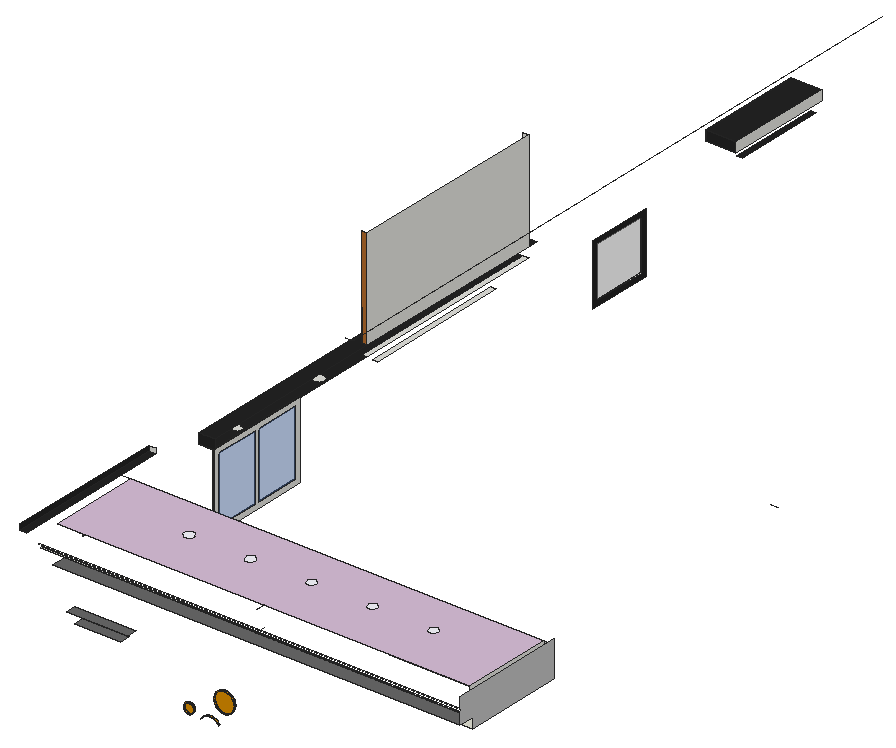
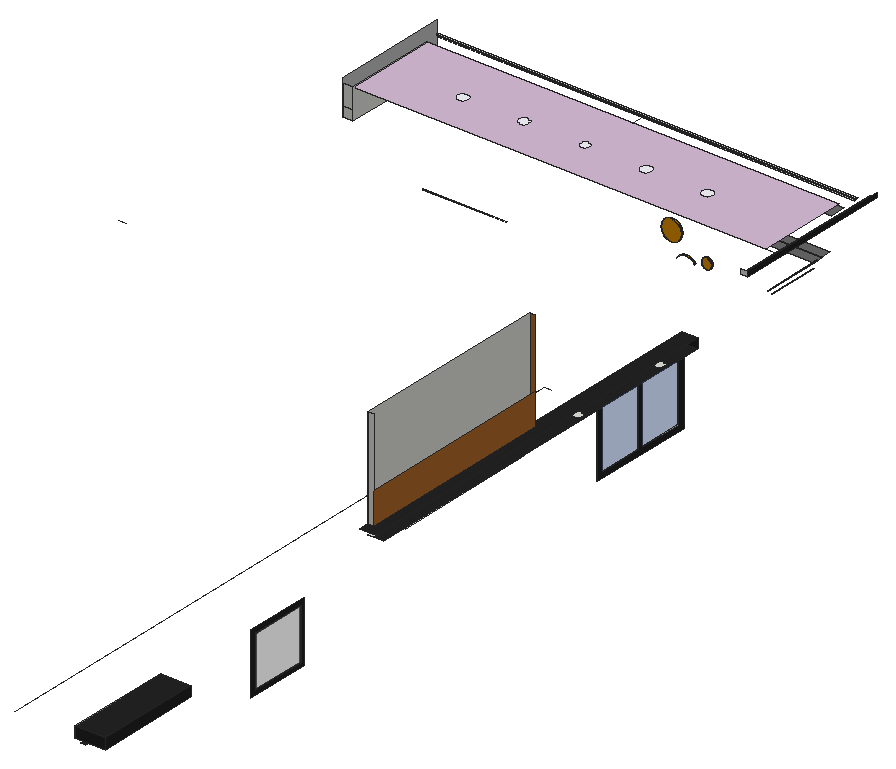
# SketchUp Ruby script. Lengths in inches.
U = 1.inch
M = Sketchup.active_model
def pt(a) = Geom::Point3d.new(a.map { |v| v * U })
def face(e, loops, mat)
  f = e.add_face(loops[0].map { |a| pt(a) })
  loops[1..].each { |l| e.add_face(l.map { |a| pt(a) }).erase! }
  f.material = f.back_material = mat if mat
  f
end
# faces: each face lists its corners as indices into pts; further lists are holes
def faces(e, pts, list, mat = nil) = list.each { |f| face(e, (f[0].is_a?(Array) ? f : [f]).map { |l| l.map { |i| pts[i] } }, mat) }
# xy, xz, yz: faces in a plane at the given z, y or x. An outline is a flat list of corners, or four numbers for a rectangle; further outlines are holes
def ring(l) = l.size == 4 ? [[l[0], l[1]], [l[2], l[1]], [l[2], l[3]], [l[0], l[3]]] : l.each_slice(2).to_a
def flat(e, list, mat, &to3) = list.each { |f| face(e, (f[0].is_a?(Array) ? f : [f]).map { |l| ring(l).map { |u, v| to3.(u, v) } }, mat) }
def xy(e, z, list, mat = nil) = flat(e, list, mat) { |x, y| [x, y, z] }
def xz(e, y, list, mat = nil) = flat(e, list, mat) { |x, z| [x, y, z] }
def yz(e, x, list, mat = nil) = flat(e, list, mat) { |y, z| [x, y, z] }
def lines(e, pts, list) = list.each { |a, b| e.add_line(pt(pts[a]), pt(pts[b])) }
# prism: a flat outline (further loops are holes) pulled along v
def prism(e, loops, v, mat = nil)
  f = face(e, loops, mat); d = Geom::Vector3d.new(v.map { |x| x * U })
  f.pushpull(f.normal.samedirection?(d) ? d.length : -d.length)
end
def box(e, o, s, mat = nil) = prism(e, [[o, [o[0] + s[0], o[1], o[2]], [o[0] + s[0], o[1] + s[1], o[2]], [o[0], o[1] + s[1], o[2]]]], [0, 0, s[2]], mat)
def at(x, y, z, deg = 0) = Geom::Transformation.translation(pt([x, y, z])) * Geom::Transformation.rotation(ORIGIN, Z_AXIS, deg.degrees)
def axes(o, x, y, z) = Geom::Transformation.new([*x, 0, *y, 0, *z, 0, *pt(o).to_a, 1])
def part(name) = M.definitions.add(name)
# library, detail: a bought-in or finely detailed component or shape, given as its bounding box
def library(name, o, s) = part(name).tap { |d| box(d.entities, o, s) }
def detail(e, o, s) = box(e.add_group.entities, o, s)
def put(e, d, t, mat = nil) = e.add_instance(d, t).tap { |i| i.material = mat if mat }
def group(e, t, mat = nil) = e.add_group.tap { |g| g.transformation = t; g.material = mat if mat }.entities
root = M.entities
M.materials.add("[0038_Orange]").color = [221, 143, 0]
M.materials.add("[0053_Ivory]").color = [255, 255, 240]
M.materials.add("[0117_GhostWhite]").color = [248, 248, 255]
M.materials.add("[0118_Thistle]").color = [216, 191, 216]
M.materials.add("[0131_Silver]").color = [192, 192, 192]
M.materials.add("[0134_DimGray]").color = [105, 105, 105]
M.materials.add("[0135_DarkGray]").color = [35, 35, 35]
M.materials.add("[Translucent Glass Blue]").color = [73, 109, 173]
M.materials["[Translucent Glass Blue]"].alpha = 0.5
M.materials.add("[Translucent Glass Gray]").color = [163, 163, 163]
M.materials["[Translucent Glass Gray]"].alpha = 0.5
M.materials.add("[Wood Bamboo]").color = [177, 105, 43]
xy(root,735.4,[[70,1678.125,72,1810.125]])
xy(root,735.4,[[69,552,72,804]],"[0135_DarkGray]")
xy(root,744.7,[[513.45,27,515.96,30]],"[0038_Orange]")
xy(root,747.4,[[69,564,72,673],[69,683,72,792]],"[0135_DarkGray]")
xy(root,822,[[174,12,282,36]],"[0134_DimGray]")
xy(root,827.4375,[[705.53,276,902.41,278]])
xy(root,840,[[156,12,300,36]],"[0134_DimGray]")
xy(root,849.4,[[60,2106,72,2322]],"[0135_DarkGray]")
xy(root,855.4,[[70,1678.125,72,1810.125]])
xy(root,867.4,[[60,2088,72,2340],[30,2202,28.75,2202.07,27.51,2202.26,26.29,2202.59,25.12,2203.04,24,2203.61,22.95,2204.29,21.97,2205.08,21.08,2205.97,20.29,2206.95,19.61,2208,19.04,2209.12,18.59,2210.29,18.26,2211.51,18.07,2212.75,18,2214,18.07,2215.25,18.26,2216.49,18.59,2217.71,19.04,2218.88,19.61,2220,20.29,2221.05,21.08,2222.03,21.97,2222.92,22.95,2223.71,24,2224.39,25.12,2224.96,26.29,2225.41,27.51,2225.74,28.75,2225.93,30,2226,31.25,2225.93,32.49,2225.74,33.71,2225.41,34.88,2224.96,36,2224.39,37.05,2223.71,38.03,2222.92,38.92,2222.03,39.71,2221.05,40.39,2220,40.96,2218.88,41.41,2217.71,41.74,2216.49,41.93,2215.25,42,2214,41.93,2212.75,41.74,2211.51,41.41,2210.29,40.96,2209.12,40.39,2208,39.71,2206.95,38.92,2205.97,38.03,2205.08,37.05,2204.29,36,2203.61,34.88,2203.04,33.71,2202.59,32.49,2202.26,31.25,2202.07]])
xy(root,867.4,[[[0,2088,60,2340],[30,2202,31.25,2202.07,32.49,2202.26,33.71,2202.59,34.88,2203.04,36,2203.61,37.05,2204.29,38.03,2205.08,38.92,2205.97,39.71,2206.95,40.39,2208,40.96,2209.12,41.41,2210.29,41.74,2211.51,41.93,2212.75,42,2214,41.93,2215.25,41.74,2216.49,41.41,2217.71,40.96,2218.88,40.39,2220,39.71,2221.05,38.92,2222.03,38.03,2222.92,37.05,2223.71,36,2224.39,34.88,2224.96,33.71,2225.41,32.49,2225.74,31.25,2225.93,30,2226,28.75,2225.93,27.51,2225.74,26.29,2225.41,25.12,2224.96,24,2224.39,22.95,2223.71,21.97,2222.92,21.08,2222.03,20.29,2221.05,19.61,2220,19.04,2218.88,18.59,2217.71,18.26,2216.49,18.07,2215.25,18,2214,18.07,2212.75,18.26,2211.51,18.59,2210.29,19.04,2209.12,19.61,2208,20.29,2206.95,21.08,2205.97,21.97,2205.08,22.95,2204.29,24,2203.61,25.12,2203.04,26.29,2202.59,27.51,2202.26,28.75,2202.07]]],"[0135_DarkGray]")
xy(root,891.4,[[60,1032,72,1380]])
xy(root,891.4,[[0,2088,72,2340]],"[0135_DarkGray]")
xy(root,903.4,[[69,167.11,72,287.92],[69,564,72,673],[69,683,72,792]],"[0135_DarkGray]")
xy(root,912,[[582,36,582,60,1068,60,1068,276,1092,276,1092,36]])
xy(root,915.4,[[69,552,72,804],[52.84,630.27,51.59,630.38,50.36,630.62,49.16,630.99,48,631.48,46.9,632.09,45.875,632.81,44.93,633.64,44.07,634.56,43.32,635.56,42.67,636.64,42.14,637.78,41.74,638.97,41.46,640.19,41.31,641.44,41.29,642.7,41.4,643.95,41.64,645.18,42.01,646.38,42.5,647.54,43.11,648.63,43.83,649.66,44.66,650.61,45.58,651.46,46.58,652.22,47.66,652.86,48.8,653.39,49.99,653.8,51.21,654.08,52.46,654.23,53.72,654.25,54.97,654.14,56.2,653.9,57.4,653.53,58.55,653.04,59.65,652.43,60.68,651.7,61.625,650.88,62.48,649.96,63.24,648.95,63.88,647.875,64.41,646.74,64.82,645.55,65.1,644.32,65.25,643.08,65.27,641.82,65.16,640.57,64.92,639.34,64.55,638.14,64.05,636.98,63.44,635.88,62.72,634.86,61.9,633.91,60.98,633.05,59.97,632.3,58.89,631.66,57.76,631.125,56.57,630.72,55.34,630.4375,54.1,630.29],[52.84,870.64,51.59,870.75,50.36,871,49.16,871.36,48,871.86,46.9,872.47,45.875,873.19,44.93,874.02,44.07,874.94,43.32,875.94,42.67,877.02,42.14,878.16,41.74,879.34,41.46,880.57,41.31,881.82,41.29,883.07,41.4,884.32,41.64,885.56,42.01,886.76,42.5,887.91,43.11,889.01,43.83,890.04,44.66,890.98,45.58,891.84,46.58,892.59,47.66,893.24,48.8,893.77,49.99,894.17,51.21,894.46,52.46,894.61,53.72,894.625,54.97,894.51,56.2,894.27,57.4,893.9,58.55,893.41,59.65,892.8,60.68,892.08,61.625,891.25,62.48,890.33,63.24,889.33,63.88,888.25,64.41,887.11,64.82,885.92,65.1,884.7,65.25,883.45,65.27,882.2,65.16,880.95,64.92,879.71,64.55,878.51,64.05,877.36,63.44,876.26,62.72,875.23,61.9,874.28,60.98,873.43,59.97,872.68,58.89,872.03,57.76,871.5,56.57,871.09,55.34,870.8125,54.1,870.66],[60,1000.8,72,1476]])
xy(root,915.4,[[69,155.11,72,299.92],[[36,552,36,1476,60,1476,60,1000.8,72,1000.8,72,804,69,804,69,552],[52.84,870.64,54.1,870.66,55.34,870.8125,56.57,871.09,57.76,871.5,58.89,872.03,59.97,872.68,60.98,873.43,61.9,874.28,62.72,875.23,63.44,876.26,64.05,877.36,64.55,878.51,64.92,879.71,65.16,880.95,65.27,882.2,65.25,883.45,65.1,884.7,64.82,885.92,64.41,887.11,63.88,888.25,63.24,889.33,62.48,890.33,61.625,891.25,60.68,892.08,59.65,892.8,58.55,893.41,57.4,893.9,56.2,894.27,54.97,894.51,53.72,894.625,52.46,894.61,51.21,894.46,49.99,894.17,48.8,893.77,47.66,893.24,46.58,892.59,45.58,891.84,44.66,890.98,43.83,890.04,43.11,889.01,42.5,887.91,42.01,886.76,41.64,885.56,41.4,884.32,41.29,883.07,41.31,881.82,41.46,880.57,41.74,879.34,42.14,878.16,42.67,877.02,43.32,875.94,44.07,874.94,44.93,874.02,45.875,873.19,46.9,872.47,48,871.86,49.16,871.36,50.36,871,51.59,870.75],[52.84,630.27,54.1,630.29,55.34,630.4375,56.57,630.72,57.76,631.125,58.89,631.66,59.97,632.3,60.98,633.05,61.9,633.91,62.72,634.86,63.44,635.88,64.05,636.98,64.55,638.14,64.92,639.34,65.16,640.57,65.27,641.82,65.25,643.08,65.1,644.32,64.82,645.55,64.41,646.74,63.88,647.875,63.24,648.95,62.48,649.96,61.625,650.88,60.68,651.7,59.65,652.43,58.55,653.04,57.4,653.53,56.2,653.9,54.97,654.14,53.72,654.25,52.46,654.23,51.21,654.08,49.99,653.8,48.8,653.39,47.66,652.86,46.58,652.22,45.58,651.46,44.66,650.61,43.83,649.66,43.11,648.63,42.5,647.54,42.01,646.38,41.64,645.18,41.4,643.95,41.29,642.7,41.31,641.44,41.46,640.19,41.74,638.97,42.14,637.78,42.67,636.64,43.32,635.56,44.07,634.56,44.93,633.64,45.875,632.81,46.9,632.09,48,631.48,49.16,630.99,50.36,630.62,51.59,630.38]]],"[0135_DarkGray]")
xy(root,936,[[132,0,1092,36]],"[0134_DimGray]")
xy(root,939.4,[[60,1000.8,72,1476]])
xy(root,939.4,[[36,552,72,552,72,1000.8,60,1000.8,60,1476,72,1476,72,1500,36,1500]],"[0135_DarkGray]")
xy(root,963,[[105,0,1092,3]])
xy(root,969,[[99,0,1092,3]])
xy(root,984,[[310.43,167.36,307.32,167.77,304.43,168.97,301.94,170.88,300.04,173.36,298.84,176.26,298.43,179.36,298.84,182.47,300.04,185.36,301.94,187.85,304.43,189.75,307.32,190.95,310.43,191.36,313.53,190.95,316.43,189.75,318.91,187.85,320.82,185.36,322.02,182.47,322.43,179.36,322.02,176.26,320.82,173.36,318.91,170.88,316.43,168.97,313.53,167.77],[454.43,167.36,451.32,167.77,448.43,168.97,445.94,170.88,444.04,173.36,442.84,176.26,442.43,179.36,442.84,182.47,444.04,185.36,445.94,187.85,448.43,189.75,451.32,190.95,454.43,191.36,457.53,190.95,460.43,189.75,462.91,187.85,464.82,185.36,466.02,182.47,466.43,179.36,466.02,176.26,464.82,173.36,462.91,170.88,460.43,168.97,457.53,167.77],[598.43,167.36,595.32,167.77,592.43,168.97,589.94,170.88,588.04,173.36,586.84,176.26,586.43,179.36,586.84,182.47,588.04,185.36,589.94,187.85,592.43,189.75,595.32,190.95,598.43,191.36,601.53,190.95,604.43,189.75,606.91,187.85,608.82,185.36,610.02,182.47,610.43,179.36,610.02,176.26,608.82,173.36,606.91,170.88,604.43,168.97,601.53,167.77],[742.43,167.36,739.32,167.77,736.43,168.97,733.94,170.88,732.04,173.36,730.84,176.26,730.43,179.36,730.84,182.47,732.04,185.36,733.94,187.85,736.43,189.75,739.32,190.95,742.43,191.36,745.53,190.95,748.43,189.75,750.91,187.85,752.82,185.36,754.02,182.47,754.43,179.36,754.02,176.26,752.82,173.36,750.91,170.88,748.43,168.97,745.53,167.77],[886.43,167.36,883.32,167.77,880.43,168.97,877.94,170.88,876.04,173.36,874.84,176.26,874.43,179.36,874.84,182.47,876.04,185.36,877.94,187.85,880.43,189.75,883.32,190.95,886.43,191.36,889.53,190.95,892.43,189.75,894.91,187.85,896.82,185.36,898.02,182.47,898.43,179.36,898.02,176.26,896.82,173.36,894.91,170.88,892.43,168.97,889.53,167.77]],"[0117_GhostWhite]")
xy(root,984,[[[96,60,1068,276],[742.43,167.36,745.53,167.77,748.43,168.97,750.91,170.88,752.82,173.36,754.02,176.26,754.43,179.36,754.02,182.47,752.82,185.36,750.91,187.85,748.43,189.75,745.53,190.95,742.43,191.36,739.32,190.95,736.43,189.75,733.94,187.85,732.04,185.36,730.84,182.47,730.43,179.36,730.84,176.26,732.04,173.36,733.94,170.88,736.43,168.97,739.32,167.77],[598.43,167.36,601.53,167.77,604.43,168.97,606.91,170.88,608.82,173.36,610.02,176.26,610.43,179.36,610.02,182.47,608.82,185.36,606.91,187.85,604.43,189.75,601.53,190.95,598.43,191.36,595.32,190.95,592.43,189.75,589.94,187.85,588.04,185.36,586.84,182.47,586.43,179.36,586.84,176.26,588.04,173.36,589.94,170.88,592.43,168.97,595.32,167.77],[454.43,167.36,457.53,167.77,460.43,168.97,462.91,170.88,464.82,173.36,466.02,176.26,466.43,179.36,466.02,182.47,464.82,185.36,462.91,187.85,460.43,189.75,457.53,190.95,454.43,191.36,451.32,190.95,448.43,189.75,445.94,187.85,444.04,185.36,442.84,182.47,442.43,179.36,442.84,176.26,444.04,173.36,445.94,170.88,448.43,168.97,451.32,167.77],[310.43,167.36,313.53,167.77,316.43,168.97,318.91,170.88,320.82,173.36,322.02,176.26,322.43,179.36,322.02,182.47,320.82,185.36,318.91,187.85,316.43,189.75,313.53,190.95,310.43,191.36,307.32,190.95,304.43,189.75,301.94,187.85,300.04,185.36,298.84,182.47,298.43,179.36,298.84,176.26,300.04,173.36,301.94,170.88,304.43,168.97,307.32,167.77],[886.43,167.36,889.53,167.77,892.43,168.97,894.91,170.88,896.82,173.36,898.02,176.26,898.43,179.36,898.02,182.47,896.82,185.36,894.91,187.85,892.43,189.75,889.53,190.95,886.43,191.36,883.32,190.95,880.43,189.75,877.94,187.85,876.04,185.36,874.84,182.47,874.43,179.36,874.84,176.26,876.04,173.36,877.94,170.88,880.43,168.97,883.32,167.77]]],"[0118_Thistle]")
xy(root,984,[[56,0,72,378]],"[0135_DarkGray]")
xz(root,30,[[432.01,715.13,433.26,715.26,434.49,715.51,435.6875,715.89,436.84,716.4,437.93,717.02,438.95,717.75,439.89,718.59,440.73,719.52,441.48,720.53,442.11,721.61,442.63,722.76,443.02,723.95,443.29,725.18,443.43,726.42,443.4375,727.68,443.3125,728.93,443.06,730.16,442.68,731.36,442.17,732.51,441.55,733.6,440.82,734.62,439.98,735.56,439.05,736.4,438.04,737.15,436.96,737.78,435.8125,738.3,434.62,738.69,433.39,738.96,432.15,739.1,430.89,739.11,429.64,738.98,428.41,738.73,427.21,738.35,426.0625,737.84,424.97,737.22,423.95,736.49,423.01,735.65,422.17,734.72,421.42,733.71,420.79,732.63,420.27,731.48,419.875,730.29,419.61,729.06,419.47,727.82,419.46,726.56,419.59,725.31,419.84,724.08,420.22,722.88,420.73,721.73,421.35,720.64,422.08,719.62,422.92,718.68,423.85,717.84,424.86,717.09,425.94,716.46,427.09,715.94,428.28,715.55,429.51,715.28,430.75,715.14],[513.45,744.7,515.96,744.7,518.46,744.96,520.92,745.48,523.31,746.26,525.6,747.28,527.78,748.53,529.82,750.01,531.68,751.68,533.37,753.55,534.84,755.58,536.1,757.76,537.125,760.05,537.9,762.4375,538.43,764.9,538.69,767.39,538.69,769.91,538.43,772.4,537.91,774.86,537.14,777.25,536.12,779.55,534.86,781.72,533.39,783.76,531.71,785.625,529.85,787.31,527.8125,788.79,525.64,790.04,523.35,791.07,520.96,791.85,518.5,792.37,516,792.63,513.49,792.64,510.99,792.375,508.53,791.86,506.14,791.08,503.85,790.0625,501.67,788.81,499.64,787.33,497.77,785.65,496.09,783.79,494.61,781.76,493.35,779.58,492.33,777.29,491.55,774.9,491.02,772.44,490.76,769.94,490.76,767.43,491.02,764.93,491.54,762.48,492.3125,760.09,493.33,757.79,494.59,755.61,496.0625,753.58,497.74,751.71,499.61,750.03,501.64,748.55,503.8125,747.29,506.11,746.27,508.5,745.49,510.95,744.97]],"[0038_Orange]")
xz(root,36,[[582,912,1092,936]],"[0053_Ivory]")
xz(root,276,[[1068,912,1092,936],[1068,936,1092,984]])
xz(root,378,[[56,984,72,996]])
xz(root,552,[[69,735.4,72,915.4],[36,915.4,72,939.4]],"[0135_DarkGray]")
xz(root,564,[[69,747.4,72,903.4]],"[0135_DarkGray]")
xz(root,673,[[69,747.4,72,903.4]],"[0135_DarkGray]")
xz(root,683,[[69,747.4,72,903.4]],"[0135_DarkGray]")
xz(root,792,[[69,747.4,72,903.4]],"[0135_DarkGray]")
xz(root,804,[[69,735.4,72,915.4]],"[0135_DarkGray]")
xz(root,1000.8,[[60,939.4,72,1176]],"[Wood Bamboo]")
xz(root,1476,[[60,939.4,72,1176]])
xz(root,1678.125,[[70,735.4,72,855.4]])
xz(root,1810.125,[[70,735.4,72,855.4]])
xz(root,2088,[[0,867.4,72,891.4]],"[0135_DarkGray]")
xz(root,2340,[[0,867.4,72,891.4]],"[0135_DarkGray]")
yz(root,0,[[2088,867.4,2340,891.4]],"[0135_DarkGray]")
yz(root,56,[[0,984,378,996]],"[0135_DarkGray]")
yz(root,60,[[1000.8,939.4,1476,1014]],"[Wood Bamboo]")
yz(root,69,[[[552,735.4,804,915.4],[683,747.4,792,903.4],[564,747.4,673,903.4]]],"[0135_DarkGray]")
yz(root,70,[[1678.125,735.4,1810.125,855.4]],"[Translucent Glass Gray]")
yz(root,72,[[[552,735.4,804,915.4],[683,747.4,792,903.4],[564,747.4,673,903.4]],[2088,867.4,2340,891.4],[1000.8,939.4,1476,1176]])
yz(root,72,[[[1666.125,723.4,1822.125,867.4],[1678.125,735.4,1810.125,855.4]]],"[0135_DarkGray]")
yz(root,72,[[564,747.4,673,903.4],[683,747.4,792,903.4]],"[Translucent Glass Blue]")
yz(root,490.76,[[27,767.43,30,769.94]],"[0038_Orange]")
yz(root,538.69,[[27,767.39,30,769.91]],"[0038_Orange]")
yz(root,1068,[[60,912,276,984]])
yz(root,1092,[[36,912,276,912,276,996,0,996,0,969,3,969,3,963,0,963,0,936,36,936]],"[0131_Silver]")
p = [[460.79,27,716.96],[459.45,27,714.83],[459.45,30,714.83],[460.79,30,716.96],[429.51,27,715.28],[430.75,27,715.14],
  [430.75,30,715.14],[429.51,30,715.28],[432.01,27,715.13],[432.01,30,715.13],[433.26,27,715.26],[433.26,30,715.26],
  [428.28,27,715.55],[428.28,30,715.55],[434.49,27,715.51],[434.49,30,715.51],[501.02,27,715.43],[499.62,27,717.52],
  [499.62,30,717.52],[501.02,30,715.43],[427.09,27,715.94],[427.09,30,715.94],[435.6875,27,715.89],[435.6875,30,715.89],
  [425.94,27,716.46],[425.94,30,716.46],[436.84,27,716.4],[436.84,30,716.4],[437.93,27,717.02],[437.93,30,717.02],
  [424.86,27,717.09],[424.86,30,717.09],[438.95,27,717.75],[438.95,30,717.75],[462.34,27,718.93],[462.34,30,718.93],
  [423.85,27,717.84],[423.85,30,717.84],[498.01,27,719.45],[498.01,30,719.45],[422.92,27,718.68],[422.92,30,718.68],
  [439.89,27,718.59],[439.89,30,718.59],[440.73,27,719.52],[440.73,30,719.52],[422.08,27,719.62],[422.08,30,719.62],
  [464.09,27,720.73],[464.09,30,720.73],[496.21,27,721.2],[496.21,30,721.2],[441.48,27,720.53],[441.48,30,720.53],
  [421.35,27,720.64],[421.35,30,720.64],[442.11,27,721.61],[442.11,30,721.61],[420.73,27,721.73],[420.73,30,721.73],
  [466.02,27,722.34],[466.02,30,722.34],[494.23,27,722.75],[494.23,30,722.75],[442.63,27,722.76],[442.63,30,722.76],
  [420.22,27,722.88],[420.22,30,722.88],[468.11,27,723.74],[468.11,30,723.74],[492.11,27,724.09],[492.11,30,724.09],
  [443.02,27,723.95],[443.02,30,723.95],[419.84,27,724.08],[419.84,30,724.08],[470.33,27,724.91],[470.33,30,724.91],
  [443.29,27,725.18],[443.29,30,725.18],[419.59,27,725.31],[419.59,30,725.31],[489.85,27,725.19],[489.85,30,725.19],
  [472.66,27,725.85],[472.66,30,725.85],[443.43,27,726.42],[443.43,30,726.42],[487.49,27,726.0625],[487.49,30,726.0625],
  [419.46,27,726.56],[419.46,30,726.56],[475.08,27,726.53],[475.08,30,726.53],[485.06,27,726.68],[485.06,30,726.68],
  [443.4375,27,727.68],[443.4375,30,727.68],[477.55,27,726.96],[477.55,30,726.96],[419.47,27,727.82],[419.47,30,727.82],
  [482.57,27,727.03],[482.57,30,727.03],[480.06,27,727.13],[480.06,30,727.13],[443.3125,27,728.93],[443.3125,30,728.93],
  [419.61,27,729.06],[419.61,30,729.06],[443.06,27,730.16],[443.06,30,730.16],[419.875,27,730.29],[419.875,30,730.29],
  [442.68,27,731.36],[442.68,30,731.36],[420.27,27,731.48],[420.27,30,731.48],[442.17,27,732.51],[442.17,30,732.51],
  [420.79,27,732.63],[420.79,30,732.63],[441.55,27,733.6],[441.55,30,733.6],[421.42,27,733.71],[421.42,30,733.71],
  [440.82,27,734.62],[440.82,30,734.62],[422.17,27,734.72],[422.17,30,734.72],[439.98,27,735.56],[439.98,30,735.56],
  [423.01,27,735.65],[423.01,30,735.65],[439.05,27,736.4],[439.05,30,736.4],[423.95,27,736.49],[423.95,30,736.49],
  [438.04,27,737.15],[438.04,30,737.15],[424.97,27,737.22],[424.97,30,737.22],[436.96,27,737.78],[436.96,30,737.78],
  [426.0625,27,737.84],[426.0625,30,737.84],[427.21,27,738.35],[427.21,30,738.35],[435.8125,27,738.3],[435.8125,30,738.3],
  [428.41,27,738.73],[428.41,30,738.73],[434.62,27,738.69],[434.62,30,738.69],[429.64,27,738.98],[429.64,30,738.98],
  [433.39,27,738.96],[433.39,30,738.96],[430.89,27,739.11],[430.89,30,739.11],[432.15,27,739.1],[432.15,30,739.1],
  [510.95,27,744.97],[513.45,27,744.7],[513.45,30,744.7],[510.95,30,744.97],[515.96,27,744.7],[518.46,27,744.96],
  [518.46,30,744.96],[515.96,30,744.7],[508.5,27,745.49],[508.5,30,745.49],[520.92,27,745.48],[520.92,30,745.48],
  [506.11,27,746.27],[506.11,30,746.27],[523.31,27,746.26],[523.31,30,746.26],[503.8125,27,747.29],[503.8125,30,747.29],
  [525.6,27,747.28],[525.6,30,747.28],[501.64,27,748.55],[501.64,30,748.55],[527.78,27,748.53],[527.78,30,748.53],
  [529.82,27,750.01],[529.82,30,750.01],[499.61,27,750.03],[499.61,30,750.03],[497.74,27,751.71],[497.74,30,751.71],
  [531.68,27,751.68],[531.68,30,751.68],[496.0625,27,753.58],[496.0625,30,753.58],[533.37,27,753.55],[533.37,30,753.55],
  [494.59,27,755.61],[494.59,30,755.61],[534.84,27,755.58],[534.84,30,755.58],[493.33,27,757.79],[493.33,30,757.79],
  [536.1,27,757.76],[536.1,30,757.76],[492.3125,27,760.09],[492.3125,30,760.09],[537.125,27,760.05],[537.125,30,760.05],
  [537.9,27,762.4375],[537.9,30,762.4375],[491.54,27,762.48],[491.54,30,762.48],[538.43,27,764.9],[538.43,30,764.9],
  [491.02,27,764.93],[491.02,30,764.93],[490.76,27,767.43],[490.76,30,767.43],[538.69,27,767.39],[538.69,30,767.39],
  [491.02,27,772.44],[490.76,27,769.94],[490.76,30,769.94],[491.02,30,772.44],[538.69,27,769.91],[538.43,27,772.4],
  [538.43,30,772.4],[538.69,30,769.91],[491.55,27,774.9],[491.55,30,774.9],[537.91,27,774.86],[537.91,30,774.86],
  [492.33,27,777.29],[492.33,30,777.29],[537.14,27,777.25],[537.14,30,777.25],[493.35,27,779.58],[493.35,30,779.58],
  [536.12,27,779.55],[536.12,30,779.55],[534.86,27,781.72],[534.86,30,781.72],[494.61,27,781.76],[494.61,30,781.76],
  [533.39,27,783.76],[533.39,30,783.76],[496.09,27,783.79],[496.09,30,783.79],[497.77,27,785.65],[497.77,30,785.65],
  [531.71,27,785.625],[531.71,30,785.625],[529.85,27,787.31],[529.85,30,787.31],[499.64,27,787.33],[499.64,30,787.33],
  [501.67,27,788.81],[501.67,30,788.81],[527.8125,27,788.79],[527.8125,30,788.79],[503.85,27,790.0625],[503.85,30,790.0625],
  [525.64,27,790.04],[525.64,30,790.04],[523.35,27,791.07],[523.35,30,791.07],[506.14,27,791.08],[506.14,30,791.08],
  [508.53,27,791.86],[508.53,30,791.86],[520.96,27,791.85],[520.96,30,791.85],[518.5,27,792.37],[518.5,30,792.37],
  [510.99,27,792.375],[510.99,30,792.375],[513.49,27,792.64],[513.49,30,792.64],[516,27,792.63],[516,30,792.63],
  [72,276,984],[96,276,984],[1092,936,984],[1074,936,984],[582,60,984],[582,36,984],
  [582,60,936],[582,36,936],[90,936,984],[72,936,984],[90,2478,984],[1074,2478,984],
  [1074,2496,984],[90,2496,984]]
faces(root,p,[[0,1,2,3],[4,5,6,7],[5,8,9,6],[8,10,11,9],[12,4,7,13],[10,14,15,11],[16,17,18,19],[20,12,13,21],
  [14,22,23,15],[24,20,21,25],[22,26,27,23],[26,28,29,27],[30,24,25,31],[28,32,33,29],[34,0,3,35],[36,30,31,37],
  [17,38,39,18],[40,36,37,41],[32,42,43,33],[42,44,45,43],[46,40,41,47],[48,34,35,49],[38,50,51,39],[44,52,53,45],
  [54,46,47,55],[52,56,57,53],[58,54,55,59],[60,48,49,61],[50,62,63,51],[56,64,65,57],[66,58,59,67],[68,60,61,69],
  [62,70,71,63],[64,72,73,65],[74,66,67,75],[76,68,69,77],[72,78,79,73],[80,74,75,81],[70,82,83,71],[84,76,77,85],
  [78,86,87,79],[82,88,89,83],[90,80,81,91],[92,84,85,93],[88,94,95,89],[86,96,97,87],[98,92,93,99],[100,90,91,101],
  [94,102,103,95],[104,98,99,105],[102,104,105,103],[96,106,107,97],[108,100,101,109],[106,110,111,107],[112,108,109,113],[110,114,115,111],
  [116,112,113,117],[114,118,119,115],[120,116,117,121],[118,122,123,119],[124,120,121,125],[122,126,127,123],[128,124,125,129],[126,130,131,127],
  [132,128,129,133],[130,134,135,131],[136,132,133,137],[134,138,139,135],[140,136,137,141],[138,142,143,139],[144,140,141,145],[146,144,145,147],
  [142,148,149,143],[150,146,147,151],[148,152,153,149],[154,150,151,155],[152,156,157,153],[158,154,155,159],[156,160,161,157],[160,158,159,161],
  [162,163,164,165],[166,167,168,169],[170,162,165,171],[167,172,173,168],[174,170,171,175],[172,176,177,173],[178,174,175,179],[176,180,181,177],
  [182,178,179,183],[180,184,185,181],[184,186,187,185],[188,182,183,189],[190,188,189,191],[186,192,193,187],[194,190,191,195],[192,196,197,193],
  [198,194,195,199],[196,200,201,197],[202,198,199,203],[200,204,205,201],[206,202,203,207],[204,208,209,205],[208,210,211,209],[212,206,207,213],
  [210,214,215,211],[216,212,213,217],[218,216,217,219],[214,220,221,215],[222,223,224,225],[226,227,228,229],[230,222,225,231],[227,232,233,228],
  [234,230,231,235],[232,236,237,233],[238,234,235,239],[236,240,241,237],[240,242,243,241],[244,238,239,245],[242,246,247,243],[248,244,245,249],
  [250,248,249,251],[246,252,253,247],[252,254,255,253],[256,250,251,257],[258,256,257,259],[254,260,261,255],[262,258,259,263],[260,264,265,261],
  [264,266,267,265],[268,262,263,269],[270,268,269,271],[266,272,273,267],[272,274,275,273],[276,270,271,277],[278,276,277,279],[274,280,281,275],
  [280,278,279,281]],"[0038_Orange]")
lines(root,p,[[282,283],[284,285],[286,287],[288,289],[290,291],[290,292],[293,294],[292,295]])
